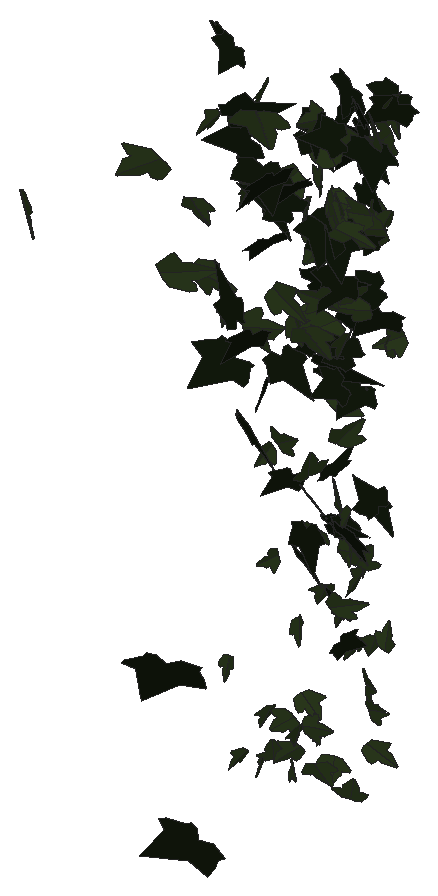
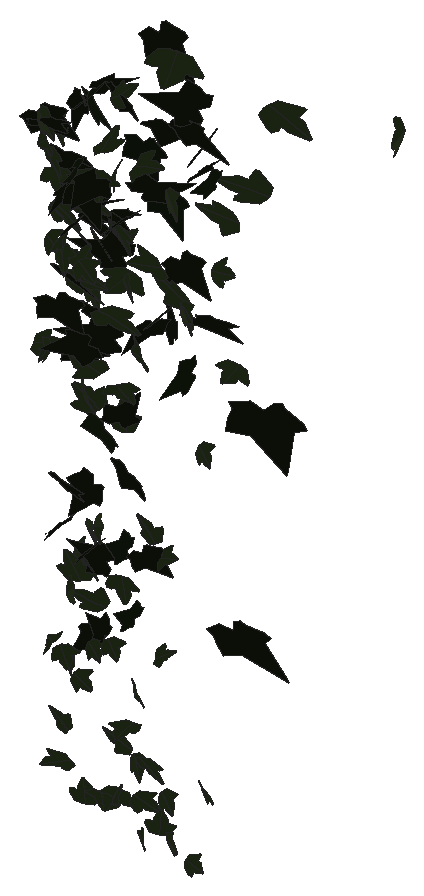
# SketchUp Ruby script. Lengths in inches.
U = 1.inch
M = Sketchup.active_model
def pt(a) = Geom::Point3d.new(a.map { |v| v * U })
def face(e, loops, mat)
  f = e.add_face(loops[0].map { |a| pt(a) })
  loops[1..].each { |l| e.add_face(l.map { |a| pt(a) }).erase! }
  f.material = f.back_material = mat if mat
  f
end
# faces: each face lists its corners as indices into pts; further lists are holes
def faces(e, pts, list, mat = nil) = list.each { |f| face(e, (f[0].is_a?(Array) ? f : [f]).map { |l| l.map { |i| pts[i] } }, mat) }
# xy, xz, yz: faces in a plane at the given z, y or x. An outline is a flat list of corners, or four numbers for a rectangle; further outlines are holes
def ring(l) = l.size == 4 ? [[l[0], l[1]], [l[2], l[1]], [l[2], l[3]], [l[0], l[3]]] : l.each_slice(2).to_a
def flat(e, list, mat, &to3) = list.each { |f| face(e, (f[0].is_a?(Array) ? f : [f]).map { |l| ring(l).map { |u, v| to3.(u, v) } }, mat) }
def xy(e, z, list, mat = nil) = flat(e, list, mat) { |x, y| [x, y, z] }
def xz(e, y, list, mat = nil) = flat(e, list, mat) { |x, z| [x, y, z] }
def yz(e, x, list, mat = nil) = flat(e, list, mat) { |y, z| [x, y, z] }
def lines(e, pts, list) = list.each { |a, b| e.add_line(pt(pts[a]), pt(pts[b])) }
# prism: a flat outline (further loops are holes) pulled along v
def prism(e, loops, v, mat = nil)
  f = face(e, loops, mat); d = Geom::Vector3d.new(v.map { |x| x * U })
  f.pushpull(f.normal.samedirection?(d) ? d.length : -d.length)
end
def box(e, o, s, mat = nil) = prism(e, [[o, [o[0] + s[0], o[1], o[2]], [o[0] + s[0], o[1] + s[1], o[2]], [o[0], o[1] + s[1], o[2]]]], [0, 0, s[2]], mat)
def at(x, y, z, deg = 0) = Geom::Transformation.translation(pt([x, y, z])) * Geom::Transformation.rotation(ORIGIN, Z_AXIS, deg.degrees)
def axes(o, x, y, z) = Geom::Transformation.new([*x, 0, *y, 0, *z, 0, *pt(o).to_a, 1])
def part(name) = M.definitions.add(name)
# library, detail: a bought-in or finely detailed component or shape, given as its bounding box
def library(name, o, s) = part(name).tap { |d| box(d.entities, o, s) }
def detail(e, o, s) = box(e.add_group.entities, o, s)
def put(e, d, t, mat = nil) = e.add_instance(d, t).tap { |i| i.material = mat if mat }
def group(e, t, mat = nil) = e.add_group.tap { |g| g.transformation = t; g.material = mat if mat }.entities
root = M.entities
M.materials.add("1026 AP 7946 SUNNY SIDE UP").color = [254, 231, 186]
M.materials.add("efeu1").color = [18, 25, 13]
M.materials.add("efeu2").color = [43, 57, 29]
c1 = part("ivyleaf_9")
p = [[1.54,2.16,1.25],[1.36,2.04,1.19],[-0.21,0.99,0.68],[-0.71,1.11,0.82],[-0.85,0.86,0.67],[-0.8,0.17,0.21],
  [-0.9,-0.01,0.1],[-0.67,-0.16,-0.02],[-0.08,-0.08,-0.05],[-0.03,-0.6,-0.4],[0.65,-0.88,-0.66],[0.83,-0.6,-0.49],
  [1.29,-0.42,-0.43],[1.8125,-0.07,-0.26],[1.21,0.44,0.15]]
faces(c1.entities,p,[[0,1,2,3,4,5,6,7,8,9,10,11,12,13,14]],"efeu1")
c2 = part("ivyleaf_10")
p = [[0,0.5,-0.03],[-0.0625,2.02,-0.43],[-0.19,2.01,-0.46],[-0.54,1.05,-0.29],[-0.52,0.625,-0.18],[-0.83,0.76,-0.28],
  [-1.16,0.64,-0.33],[-1.15,0.33,-0.24],[-0.77,-0.39,0.02],[-0.3,-0.51,0.16],[0.04,-0.48,0.23],[-0.02,2.01,-0.4375],
  [-0.06,2.01,-0.43],[0.04,-0.49,0.23],[0.67,-0.49,0.14],[1.38,0.36,-0.2],[1.375,0.51,-0.24],[0.81,0.65,-0.19],
  [0.62,0.59,-0.15],[0.6,1.09,-0.28],[0.5,1.23,-0.31]]
faces(c2.entities,p,[[0,1,2,3,4,5,6,7,8,9,10],[11,12,0,13,14,15,16,17,18,19,20]],"efeu2")
put(root,c1,axes([96.76,204.79,257.04],[0.31622,0.25415,-0.29284],[-0.24755,-0.2359,-0.34019],[-0.58798,0.236,-0.01427]),"1026 AP 7946 SUNNY SIDE UP")
put(root,c2,axes([92.11,205.87,266.17],[-0.19946,0.27307,-0.18967],[0.10139,-0.17091,-0.32043],[-0.54654,-0.13136,0.00977]),"1026 AP 7946 SUNNY SIDE UP")
put(root,c1,axes([96.56,206.05,252.18],[0.11799,0.01234,-0.4054],[-0.50602,-0.23611,-0.07008],[-0.39742,0.3043,-0.03112]),"1026 AP 7946 SUNNY SIDE UP")
put(root,c1,axes([96.82,207.04,264.5],[-0.15729,-0.25243,0.24856],[0.10943,0.22686,0.29069],[-0.57568,0.11209,-0.01265]),"1026 AP 7946 SUNNY SIDE UP")
put(root,c2,axes([93.97,207.83,266.89],[-0.32907,-0.10019,0.27299],[-0.33244,-0.17002,-0.2321],[0.32817,-0.27269,0.03861]),"1026 AP 7946 SUNNY SIDE UP")
put(root,c2,axes([94.7,207.59,264.54],[-0.15004,-0.0681,0.33403],[0.33779,0.24264,0.1201],[-0.4259,0.21643,-0.02242]),"1026 AP 7946 SUNNY SIDE UP")
put(root,c1,axes([97.24,207.8,267.68],[-0.14376,0.29444,-0.23588],[0.07304,-0.22056,-0.33064],[-0.62393,-0.09366,0.01564]),"1026 AP 7946 SUNNY SIDE UP")
put(root,c2,axes([94.8,208.48,264.21],[-0.05213,-0.01553,-0.31627],[0.4588,-0.12172,-0.02495],[-0.20331,-0.2707,0.0248]),"1026 AP 7946 SUNNY SIDE UP")
put(root,c1,axes([95.85,208.82,262.91],[-0.055,0.20258,-0.23143],[0.02728,-0.21859,-0.22226],[-0.50545,-0.03384,0.01318]),"1026 AP 7946 SUNNY SIDE UP")
put(root,c1,axes([95.07,209.17,261.92],[-0.52993,-0.11379,0.04704],[-0.05338,-0.04575,-0.35471],[0.20101,-0.31213,0.02981]),"1026 AP 7946 SUNNY SIDE UP")
put(root,c1,axes([95.87,209.09,261.23],[0.03447,0.17723,0.22376],[-0.11545,-0.1974,0.1856],[0.44754,-0.06457,0.03065]),"1026 AP 7946 SUNNY SIDE UP")
put(root,c2,axes([95.88,209.04,268.08],[-0.51085,-0.15968,-0.07554],[0.13393,-0.00356,-0.36233],[0.26277,-0.30861,0.03781]),"1026 AP 7946 SUNNY SIDE UP")
put(root,c1,axes([95.32,209.19,260.47],[0.4051,-0.21363,-0.08706],[-0.12708,0.03379,-0.34146],[0.36488,0.24895,-0.02227]),"1026 AP 7946 SUNNY SIDE UP")
put(root,c1,axes([95.69,209.4,266.63],[-0.26287,-0.20198,-0.17808],[0.20945,0.11062,-0.26953],[0.38847,-0.19632,0.02482]),"1026 AP 7946 SUNNY SIDE UP")
put(root,c2,axes([95.26,209.61,262.56],[0.21015,-0.10079,-0.30372],[0.41701,-0.14108,0.16723],[-0.29184,-0.27416,0.02025]),"1026 AP 7946 SUNNY SIDE UP")
put(root,c1,axes([95.75,209.48,264.89],[-0.01144,0.27838,-0.10004],[0.00367,-0.09705,-0.29947],[-0.50045,-0.00708,0.00009]),"1026 AP 7946 SUNNY SIDE UP")
put(root,c1,axes([95.07,209.6875,266.99],[-0.01867,-0.04256,-0.3261],[-0.49086,-0.10081,0.0249],[-0.17514,0.28706,-0.03501]),"1026 AP 7946 SUNNY SIDE UP")
put(root,c1,axes([94.79,209.64,267.48],[0.11811,0.04297,0.35046],[0.5169,0.1195,-0.08455],[-0.21422,0.31202,-0.0108]),"1026 AP 7946 SUNNY SIDE UP")
put(root,c1,axes([96.46,209.9375,257.91],[-0.26713,-0.0282,-0.2717],[0.43281,-0.01369,-0.16806],[0.0054,-0.29798,0.02923]),"1026 AP 7946 SUNNY SIDE UP")
put(root,c2,axes([96.79,210.02,263.57],[-0.12681,-0.0987,-0.24808],[-0.24998,-0.17731,0.12994],[-0.34438,0.16505,-0.00298]),"1026 AP 7946 SUNNY SIDE UP")
put(root,c1,axes([96.125,209.78,266.18],[0.03002,0.28231,-0.07055],[-0.00699,-0.06946,-0.30379],[-0.49352,0.01815,0.00001]),"1026 AP 7946 SUNNY SIDE UP")
put(root,c2,axes([95.69,209.92,263.35],[0.22264,0.02384,0.28435],[0.45215,-0.01413,-0.13981],[0.00365,0.29561,-0.02545]),"1026 AP 7946 SUNNY SIDE UP")
put(root,c2,axes([96.58,209.85,262.76],[-0.39525,-0.05768,-0.14847],[0.23823,0.00369,-0.25522],[0.0875,-0.2706,0.02422]),"1026 AP 7946 SUNNY SIDE UP")
put(root,c2,axes([96.41,210.09,259.24],[-0.13203,-0.27231,-0.09841],[-0.03041,-0.08677,0.3019],[-0.48504,0.07956,0.00786]),"1026 AP 7946 SUNNY SIDE UP")
put(root,c1,axes([95.8,209.94,261.85],[0.09352,-0.22709,-0.23612],[-0.06194,0.2148,-0.24689],[0.53029,0.06514,0.01281]),"1026 AP 7946 SUNNY SIDE UP")
put(root,c1,axes([97.09,210.2,267.47],[-0.20282,-0.05341,0.25391],[-0.29832,-0.16473,-0.1364],[0.28683,-0.20909,0.03768]),"1026 AP 7946 SUNNY SIDE UP")
put(root,c1,axes([97.07,210.28,261.49],[-0.18841,-0.12241,0.2142],[-0.16462,-0.1795,-0.17628],[0.36507,-0.14412,0.03106]),"1026 AP 7946 SUNNY SIDE UP")
put(root,c1,axes([95.76,210.1875,265.31],[-0.07196,0.0321,0.30452],[-0.48333,-0.03002,-0.04228],[0.04272,-0.2856,0.03459]),"1026 AP 7946 SUNNY SIDE UP")
put(root,c2,axes([95.77,210.35,266.05],[0.12707,0.12283,-0.29191],[-0.1913,-0.25055,-0.15655],[-0.47291,0.13435,-0.01511]),"1026 AP 7946 SUNNY SIDE UP")
put(root,c1,axes([97.15,210.27,264.12],[-0.47959,-0.0158,-0.11049],[0.17622,-0.01682,-0.30232],[0.01536,-0.30024,0.01853]),"1026 AP 7946 SUNNY SIDE UP")
put(root,c2,axes([96.33,210.43,267.59],[-0.02492,0.05935,0.29452],[0.05971,-0.27215,0.06125],[0.47271,0.03751,0.00779]),"1026 AP 7946 SUNNY SIDE UP")
put(root,c1,axes([96.32,210.4,267.64],[-0.29082,-0.01958,-0.23941],[0.38013,-0.0293,-0.18153],[-0.01944,-0.27997,0.03177]),"1026 AP 7946 SUNNY SIDE UP")
put(root,c2,axes([96.66,210.43,263.54],[0.18759,-0.1561,-0.17936],[0.20715,-0.11461,0.20137],[-0.32595,-0.16268,0.02475]),"1026 AP 7946 SUNNY SIDE UP")
put(root,c2,axes([97.09,210.45,262.6],[0.00771,-0.26051,0.02821],[0.00502,-0.0297,-0.27934],[0.44507,0.00485,0.00266]),"1026 AP 7946 SUNNY SIDE UP")
put(root,c1,axes([96.59,210.64,264.76],[-0.28307,-0.1446,-0.2224],[0.37207,0.0377,-0.21791],[0.2096,-0.26222,0.08646]),"1026 AP 7946 SUNNY SIDE UP")
put(root,c1,axes([96.27,210.44,263.65],[0.16696,0.01748,0.27789],[0.44123,-0.0051,-0.10523],[-0.00241,0.27732,-0.01557]),"1026 AP 7946 SUNNY SIDE UP")
put(root,c1,axes([96.35,210.7,264.8],[-0.24627,-0.23153,-0.02228],[0.03909,0.00653,-0.29192],[0.39226,-0.14601,0.01511]),"1026 AP 7946 SUNNY SIDE UP")
put(root,c1,axes([97.1,210.59,262.07],[-0.35743,-0.08481,-0.12875],[-0.19987,-0.02563,0.2419],[-0.1473,0.24057,-0.0158]),"1026 AP 7946 SUNNY SIDE UP")
put(root,c2,axes([96.22,210.65,264.47],[0.3782,-0.18524,-0.05736],[-0.09213,0.01449,-0.30899],[0.31295,0.22813,-0.02165]),"1026 AP 7946 SUNNY SIDE UP")
put(root,c1,axes([96.42,210.56,261.57],[0.31632,0.01269,0.2436],[0.38523,-0.03481,-0.19752],[0.03219,0.29191,-0.03]),"1026 AP 7946 SUNNY SIDE UP")
put(root,c1,axes([96.92,210.625,257.76],[0.44751,-0.04637,-0.10647],[-0.1705,-0.00169,-0.28594],[0.07268,0.28154,-0.01522]),"1026 AP 7946 SUNNY SIDE UP")
put(root,c2,axes([96.89,210.61,264.99],[-0.18325,-0.10283,-0.23851],[0.34983,0.09147,-0.15174],[0.22227,-0.22874,0.04219]),"1026 AP 7946 SUNNY SIDE UP")
put(root,c1,axes([96.7,210.49,259.17],[-0.2338,0.23128,-0.1163],[-0.07387,0.10384,0.28921],[0.42966,0.1437,-0.01356]),"1026 AP 7946 SUNNY SIDE UP")
put(root,c2,axes([97.01,210.89,263.4],[-0.12961,-0.16832,-0.16863],[-0.12959,-0.13566,0.19567],[-0.36657,0.10747,-0.00955]),"1026 AP 7946 SUNNY SIDE UP")
put(root,c1,axes([96.64,210.98,265.02],[-0.23121,-0.26511,0.07266],[0.05058,-0.09343,-0.31215],[0.46328,-0.12211,0.07034]),"1026 AP 7946 SUNNY SIDE UP")
put(root,c2,axes([96.58,210.69,265.33],[-0.02008,0.24122,0.08878],[-0.02199,0.07919,-0.25728],[-0.43073,-0.01529,0.009]),"1026 AP 7946 SUNNY SIDE UP")
put(root,c1,axes([97.03,210.97,261.13],[-0.31101,-0.19534,0.03687],[-0.02075,-0.03913,-0.28663],[0.33685,-0.18276,0.01638]),"1026 AP 7946 SUNNY SIDE UP")
put(root,c2,axes([96.78,210.73,259.89],[-0.15602,-0.22079,0.1488],[0.07236,0.13576,0.25766],[-0.43959,0.10071,-0.0104]),"1026 AP 7946 SUNNY SIDE UP")
put(root,c2,axes([96.75,210.71,260.72],[0.26225,0.07892,-0.21619],[0.28132,0.11885,0.18617],[0.23983,-0.2257,0.01803]),"1026 AP 7946 SUNNY SIDE UP")
put(root,c2,axes([96.23,210.93,262.41],[0.35497,0.029,-0.22598],[-0.34037,-0.07477,-0.2243],[-0.12419,0.28784,-0.03117]),"1026 AP 7946 SUNNY SIDE UP")
put(root,c2,axes([96.36,210.84,266.49],[0.08365,0.28964,0.04034],[-0.02287,-0.03209,0.31397],[0.4945,-0.05048,0.0077]),"1026 AP 7946 SUNNY SIDE UP")
put(root,c2,axes([96.47,210.85,265.54],[-0.00074,0.31146,-0.03662],[0.00224,-0.03826,-0.33397],[-0.53268,-0.0006,-0.00136]),"1026 AP 7946 SUNNY SIDE UP")
put(root,c2,axes([96.19,210.66,265.87],[0.00823,0.08522,-0.28036],[-0.04237,0.26209,0.09408],[0.46737,0.02226,0.01347]),"1026 AP 7946 SUNNY SIDE UP")
put(root,c2,axes([96.49,210.88,265.47],[0.09882,0.3056,-0.027],[0.0015,-0.0299,-0.3334],[-0.52113,0.05786,-0.00608]),"1026 AP 7946 SUNNY SIDE UP")
put(root,c2,axes([97.11,210.98,263.02],[-0.07467,0.00165,0.25011],[-0.32064,-0.14011,-0.03897],[0.23333,-0.19202,0.02648]),"1026 AP 7946 SUNNY SIDE UP")
put(root,c1,axes([96.68,211.06,267.6875],[-0.33881,0.13455,-0.17552],[0.20651,-0.1147,-0.25819],[-0.29773,-0.23267,0.02065]),"1026 AP 7946 SUNNY SIDE UP")
put(root,c2,axes([96.37,211,265.45],[-0.26332,0.25966,-0.05872],[0.02425,-0.05918,-0.32408],[-0.45108,-0.15476,0.01685]),"1026 AP 7946 SUNNY SIDE UP")
put(root,c2,axes([96.8,211.22,256.36],[0.0399,-0.09067,0.2451],[0.12446,-0.22498,-0.09813],[0.3813,0.08292,0.00638]),"1026 AP 7946 SUNNY SIDE UP")
put(root,c2,axes([95.02,211.27,261.91],[0.17616,-0.04264,0.27108],[0.34964,-0.15024,-0.1193],[0.26182,0.22933,-0.02308]),"1026 AP 7946 SUNNY SIDE UP")
put(root,c2,axes([96.96,211.13,265.21],[0.13555,-0.01949,-0.28992],[-0.44932,0.05607,-0.08718],[0.10068,0.27646,0.00128]),"1026 AP 7946 SUNNY SIDE UP")
put(root,c1,axes([96.45,211.4375,267.92],[-0.07216,-0.22327,0.20327],[-0.03762,-0.19181,-0.24572],[0.49933,-0.04671,0.01086]),"1026 AP 7946 SUNNY SIDE UP")
put(root,c1,axes([97.32,211.2,264.66],[-0.24554,0.17419,0.07781],[-0.09921,0.04273,-0.24113],[-0.30311,-0.15509,0.01589]),"1026 AP 7946 SUNNY SIDE UP")
put(root,c1,axes([96.75,211.22,267.74],[0.29223,-0.05908,-0.19794],[-0.30059,0.05088,-0.19401],[0.13188,0.24688,-0.00359]),"1026 AP 7946 SUNNY SIDE UP")
put(root,c2,axes([97.3125,211.3,264.88],[-0.19055,0.04583,0.23418],[-0.37648,0.00157,-0.12251],[-0.03801,-0.24533,0.03942]),"1026 AP 7946 SUNNY SIDE UP")
put(root,c1,axes([97.18,211.37,263.37],[-0.4502,0.1023,0.03345],[-0.06098,-0.01027,-0.30351],[-0.17034,-0.26669,0.02024]),"1026 AP 7946 SUNNY SIDE UP")
put(root,c2,axes([96.84,211.47,253.64],[-0.12272,0.07005,0.23584],[0.30166,-0.12505,0.10625],[0.2242,0.20659,-0.01387]),"1026 AP 7946 SUNNY SIDE UP")
put(root,c2,axes([95.34,211.43,252.14],[0.09559,-0.05032,-0.22976],[0.31746,-0.09584,0.07852],[-0.16776,-0.21005,0.01766]),"1026 AP 7946 SUNNY SIDE UP")
put(root,c2,axes([96.18,211.32,255.36],[-0.15734,-0.06078,0.22516],[0.25434,0.14891,0.11963],[-0.25084,0.1891,-0.01993]),"1026 AP 7946 SUNNY SIDE UP")
put(root,c1,axes([96.32,211.29,254.59],[-0.01301,0.02501,-0.25525],[-0.13285,0.23307,0.02849],[0.36858,0.08489,0.00126]),"1026 AP 7946 SUNNY SIDE UP")
put(root,c2,axes([94.98,211.5,251.94],[-0.00745,-0.23171,-0.01564],[0.00479,0.01381,-0.23866],[0.36496,-0.00491,0.00282]),"1026 AP 7946 SUNNY SIDE UP")
put(root,c1,axes([97.15,211.55,262.69],[0.11918,0.13233,-0.24427],[-0.14865,-0.21292,-0.16281],[-0.42505,0.11157,-0.01155]),"1026 AP 7946 SUNNY SIDE UP")
put(root,c1,axes([97.125,211.44,258.11],[-0.33665,0.00804,-0.15131],[-0.22838,0.02999,0.21991],[0.03705,0.25792,-0.01933]),"1026 AP 7946 SUNNY SIDE UP")
put(root,c1,axes([96.85,211.64,266.54],[-0.33708,-0.13563,-0.16656],[0.24213,0.06248,-0.25525],[0.25011,-0.24328,0.02263]),"1026 AP 7946 SUNNY SIDE UP")
put(root,c2,axes([94.65,211.57,252.02],[0.2905,-0.07094,-0.1166],[-0.17836,0.0174,-0.2026],[0.10991,0.21576,-0.02059]),"1026 AP 7946 SUNNY SIDE UP")
put(root,c2,axes([97.21,211.38,266.99],[-0.07274,0.09334,-0.27361],[-0.18286,0.2331,0.1132],[0.42624,0.11593,0.00187]),"1026 AP 7946 SUNNY SIDE UP")
put(root,c2,axes([96.21,211.7,260.7],[0.23048,-0.12885,0.19348],[0.19047,-0.14606,-0.2007],[0.30441,0.18895,-0.02092]),"1026 AP 7946 SUNNY SIDE UP")
put(root,c2,axes([95.17,211.49,252.73],[0.16574,0.18338,0.10562],[0.09705,0.0814,-0.2171],[-0.31495,0.12159,-0.01131]),"1026 AP 7946 SUNNY SIDE UP")
put(root,c2,axes([96.125,211.6875,257.42],[0.19705,-0.2116,0.02366],[0.00282,-0.02699,-0.2532],[0.33488,0.12474,-0.01179]),"1026 AP 7946 SUNNY SIDE UP")
put(root,c2,axes([94.65,211.78,251.2],[-0.13826,-0.11587,0.17426],[-0.10854,-0.15733,-0.14834],[0.30448,-0.1087,0.02625]),"1026 AP 7946 SUNNY SIDE UP")
put(root,c1,axes([92.93,211.87,267.51],[-0.11246,-0.20782,0.14205],[-0.06539,-0.13275,-0.22718],[0.38773,-0.08267,0.00289]),"1026 AP 7946 SUNNY SIDE UP")
put(root,c2,axes([96.21,211.73,250.65],[-0.30519,-0.08983,0.00949],[0.00726,0.01315,0.22017],[-0.14188,0.19389,-0.00915]),"1026 AP 7946 SUNNY SIDE UP")
put(root,c2,axes([95.36,211.6875,251.05],[-0.28738,-0.10428,-0.09434],[0.13639,0.03111,-0.21607],[0.16956,-0.20177,0.01392]),"1026 AP 7946 SUNNY SIDE UP")
put(root,c1,axes([95.59,211.89,255.06],[0.10301,-0.11211,0.21471],[0.119,-0.19567,-0.13367],[0.35351,0.09853,-0.01757]),"1026 AP 7946 SUNNY SIDE UP")
put(root,c1,axes([94.97,211.87,257.37],[0.22261,-0.17413,0.11388],[0.08929,-0.09724,-0.23121],[0.31265,0.15175,-0.01506]),"1026 AP 7946 SUNNY SIDE UP")
put(root,c2,axes([95.97,211.9,256.65],[0.23883,-0.09291,0.18691],[0.21845,-0.11928,-0.18291],[0.23555,0.20482,-0.01988]),"1026 AP 7946 SUNNY SIDE UP")
put(root,c1,axes([95.91,211.88,257.08],[0.11336,-0.23682,-0.0694],[-0.0355,0.06213,-0.25464],[0.38495,0.07547,-0.00305]),"1026 AP 7946 SUNNY SIDE UP")
put(root,c2,axes([96.33,211.84,256.28],[-0.33745,-0.11311,0.08436],[0.09928,0.05663,0.24943],[-0.19651,0.22284,-0.01885]),"1026 AP 7946 SUNNY SIDE UP")
put(root,c1,axes([94.67,211.97,255.8],[0.16559,-0.19279,0.10222],[0.07376,-0.08868,-0.22682],[0.33367,0.11528,-0.00059]),"1026 AP 7946 SUNNY SIDE UP")
put(root,c2,axes([93.98,211.92,250.74],[-0.205,-0.16585,-0.04292],[-0.05523,-0.02409,0.21681],[-0.26279,0.13445,-0.01208]),"1026 AP 7946 SUNNY SIDE UP")
put(root,c1,axes([97.23,211.99,267.56],[0.03011,0.05998,-0.28282],[-0.11576,-0.25604,-0.07052],[-0.44639,0.07044,-0.00079]),"1026 AP 7946 SUNNY SIDE UP")
put(root,c2,axes([93.65,211.98,250.57],[0.14133,-0.15974,0.10656],[0.06167,-0.09741,-0.189],[0.29361,0.09735,-0.0116]),"1026 AP 7946 SUNNY SIDE UP")
put(root,c1,axes([95.54,211.89,256.89],[0.26716,0.02416,-0.19098],[0.27346,0.07196,0.17416],[0.10842,-0.24105,0.0313]),"1026 AP 7946 SUNNY SIDE UP")
put(root,c2,axes([95.875,211.74,257.58],[-0.09561,0.10975,-0.21482],[-0.13571,0.19071,0.13006],[0.34572,0.10522,-0.00836]),"1026 AP 7946 SUNNY SIDE UP")
put(root,c2,axes([95.07,211.91,256.56],[-0.35446,0.00293,0.06171],[-0.09394,-0.03065,-0.23031],[0.00796,-0.23122,0.02994]),"1026 AP 7946 SUNNY SIDE UP")
put(root,c2,axes([97.21,212.09,261.88],[0.08603,0.03927,-0.2571],[-0.2261,-0.20539,-0.06691],[-0.32704,0.15232,-0.02137]),"1026 AP 7946 SUNNY SIDE UP")
put(root,c2,axes([95.8125,211.96,266.47],[-0.41858,-0.10135,0.06033],[-0.06201,-0.06097,-0.28278],[0.18799,-0.24578,0.04105]),"1026 AP 7946 SUNNY SIDE UP")
put(root,c1,axes([94.32,212.05,257.58],[-0.00429,0.08886,-0.23244],[-0.02938,-0.22555,-0.0924],[-0.3809,0.0164,0.00974]),"1026 AP 7946 SUNNY SIDE UP")
put(root,c2,axes([93.625,212.02,266.73],[0.08552,-0.25123,0.00762],[-0.00201,-0.0093,-0.26485],[0.39528,0.05431,-0.00299]),"1026 AP 7946 SUNNY SIDE UP")
put(root,c2,axes([95.49,212.01,251.09],[0.33656,0.02654,0.02645],[0.04347,-0.01642,-0.22137],[-0.03824,0.21493,-0.01889]),"1026 AP 7946 SUNNY SIDE UP")
put(root,c2,axes([92.17,212.16,265.43],[0.031,-0.115,0.22397],[0.02669,-0.2176,-0.12107],[0.38671,0.02424,-0.0096]),"1026 AP 7946 SUNNY SIDE UP")
put(root,c2,axes([94.46,212.1,254.04],[0.19238,-0.08379,0.18368],[0.2115,-0.11858,-0.15279],[0.22726,0.18129,-0.0133]),"1026 AP 7946 SUNNY SIDE UP")
put(root,c2,axes([92.96,212.125,250.35],[-0.00557,-0.14778,0.14293],[-0.00061,-0.1396,-0.15309],[0.31964,-0.00284,0.0022]),"1026 AP 7946 SUNNY SIDE UP")
put(root,c2,axes([93.72,212.07,251.7],[-0.02684,-0.20834,0.05577],[-0.00474,-0.05526,-0.21567],[0.33892,-0.01727,0.0014]),"1026 AP 7946 SUNNY SIDE UP")
put(root,c2,axes([95.95,212.15,264.25],[-0.12599,-0.19384,0.11935],[-0.01953,-0.12011,-0.21455],[0.35544,-0.07531,0.03052]),"1026 AP 7946 SUNNY SIDE UP")
put(root,c1,axes([96.04,212.01,266.05],[0.0564,0.23522,-0.13262],[-0.05552,-0.12338,-0.25564],[-0.45033,0.04467,0.01491]),"1026 AP 7946 SUNNY SIDE UP")
put(root,c2,axes([95.71,212.13,254.8],[-0.03097,-0.18887,0.07854],[0.00947,-0.07818,-0.19563],[0.32076,-0.01593,0.01336]),"1026 AP 7946 SUNNY SIDE UP")
put(root,c2,axes([94.25,212.17,250.43],[0.013,0.01026,0.20843],[0.24146,-0.1323,-0.00032],[0.20762,0.15322,-0.01267]),"1026 AP 7946 SUNNY SIDE UP")
put(root,c2,axes([96.56,212.1,254.39],[-0.17455,-0.16804,0.04654],[-0.01892,-0.04718,-0.20713],[0.27334,-0.11057,0.01539]),"1026 AP 7946 SUNNY SIDE UP")
put(root,c2,axes([97.0625,212.15,267.59],[0.06247,-0.2586,0.0719],[0.00087,-0.07112,-0.28046],[0.45501,0.03564,-0.00934]),"1026 AP 7946 SUNNY SIDE UP")
put(root,c2,axes([96.8125,212.2,264.64],[-0.01657,-0.19811,0.144],[0.06837,-0.1403,-0.20068],[0.37609,0.01677,0.04283]),"1026 AP 7946 SUNNY SIDE UP")
put(root,c2,axes([93.11,212.14,264.13],[0.08157,-0.23182,0.05317],[0.01863,-0.05159,-0.24503],[0.37344,0.05321,0.00061]),"1026 AP 7946 SUNNY SIDE UP")
put(root,c1,axes([96.03,211.94,262.16],[0.06069,0.05378,-0.26669],[0.18394,0.23149,0.06879],[0.37337,-0.12278,0.00946]),"1026 AP 7946 SUNNY SIDE UP")
put(root,c2,axes([94.67,212.19,264.22],[0.18218,-0.18488,0.1186],[0.10682,-0.09447,-0.22522],[0.32629,0.13415,0.00751]),"1026 AP 7946 SUNNY SIDE UP")
put(root,c1,axes([92.28,212.16,267.61],[0.24464,-0.20369,0.01249],[-0.0059,-0.01955,-0.26372],[0.3209,0.15492,-0.01437]),"1026 AP 7946 SUNNY SIDE UP")
put(root,c2,axes([93.73,212.25,255.3],[0.03244,0.01868,-0.2195],[-0.1279,-0.19741,-0.02708],[-0.31123,0.08307,-0.01175]),"1026 AP 7946 SUNNY SIDE UP")
put(root,c1,axes([94.9,212.19,260.78],[0.14585,0.06554,0.23065],[-0.33391,-0.07505,0.11302],[0.15048,-0.23006,0.02724]),"1026 AP 7946 SUNNY SIDE UP")
put(root,c2,axes([96.43,212.16,252.58],[-0.15837,0.04715,0.19973],[0.30056,-0.03846,0.11186],[0.08856,0.21483,-0.02245]),"1026 AP 7946 SUNNY SIDE UP")
put(root,c2,axes([96.93,212.0625,266.72],[0.24278,-0.13804,-0.15105],[-0.13448,0.12124,-0.2108],[0.28569,0.17438,0.02914]),"1026 AP 7946 SUNNY SIDE UP")
put(root,c2,axes([93.13,212.12,264.09],[0.22642,-0.18941,-0.0543],[-0.03342,0.04861,-0.24451],[0.30689,0.14504,0.01344]),"1026 AP 7946 SUNNY SIDE UP")
put(root,c2,axes([96.2,212.29,256.0625],[0.06269,-0.02943,0.23614],[0.1903,-0.1957,-0.04868],[0.30987,0.12613,-0.01788]),"1026 AP 7946 SUNNY SIDE UP")
put(root,c2,axes([93.58,212.26,257.84],[0.05324,0.11144,-0.20584],[-0.09601,-0.19092,-0.12109],[-0.3476,0.0698,0.00192]),"1026 AP 7946 SUNNY SIDE UP")
put(root,c2,axes([97.07,211.95,261.73],[-0.00181,0.03529,0.25164],[-0.14011,0.21988,-0.03274],[-0.37754,-0.08177,0.01094]),"1026 AP 7946 SUNNY SIDE UP")
put(root,c2,axes([96.54,212.12,264.41],[-0.01966,-0.24613,-0.05539],[0.0189,0.04803,-0.26296],[0.42545,-0.01351,0.00912]),"1026 AP 7946 SUNNY SIDE UP")
put(root,c2,axes([96.91,211.99,254.43],[0.06158,0.16442,-0.16566],[0.01518,0.16275,0.17379],[0.36234,-0.03476,0.02087]),"1026 AP 7946 SUNNY SIDE UP")
put(root,c2,axes([95.15,212.19,255.1],[-0.11002,-0.18275,0.05203],[-0.02021,-0.05025,-0.20181],[0.29789,-0.07091,0.00553]),"1026 AP 7946 SUNNY SIDE UP")
put(root,c1,axes([94.73,212.14,265.87],[0.13735,-0.21244,-0.11502],[-0.00994,0.11548,-0.2333],[0.37635,0.08058,0.03581]),"1026 AP 7946 SUNNY SIDE UP")
put(root,c2,axes([96.5,212.18,264.77],[-0.00242,0.24386,-0.08272],[-0.02351,-0.0804,-0.26179],[-0.43526,0.00299,0.0146]),"1026 AP 7946 SUNNY SIDE UP")
put(root,c1,axes([95.7,212.03,266.47],[0.43193,0.08296,-0.05266],[-0.0926,0.00568,-0.28547],[-0.13616,0.2593,0.02709]),"1026 AP 7946 SUNNY SIDE UP")
put(root,c1,axes([96.98,212.3,267.6],[-0.32542,-0.14515,0.03944],[-0.03025,-0.04043,-0.25969],[0.23444,-0.2067,0.02124]),"1026 AP 7946 SUNNY SIDE UP")
put(root,c1,axes([96.24,212.12,265.18],[0.16149,-0.17898,-0.1373],[-0.09169,0.11894,-0.21176],[0.33771,0.11788,0.00816]),"1026 AP 7946 SUNNY SIDE UP")
put(root,c2,axes([94.85,212.21,261.61],[0.30758,0.10907,-0.1041],[-0.12156,-0.06922,-0.23014],[-0.20049,0.20931,-0.02017]),"1026 AP 7946 SUNNY SIDE UP")
put(root,c2,axes([93.95,212.18,258.17],[-0.25662,0.03249,0.17428],[0.26629,-0.01101,0.17061],[0.04802,0.23467,-0.01472]),"1026 AP 7946 SUNNY SIDE UP")
put(root,c2,axes([96.63,212.17,266.34],[-0.36366,-0.08472,0.04733],[-0.05687,-0.03575,-0.25305],[0.14085,-0.23317,0.02003]),"1026 AP 7946 SUNNY SIDE UP")
put(root,c1,axes([96.1,212.18,266.63],[0.23961,-0.20373,-0.06768],[-0.08359,0.04064,-0.26122],[0.32547,0.16042,-0.01726]),"1026 AP 7946 SUNNY SIDE UP")
put(root,c2,axes([92.48,212.24,252.37],[0.23636,-0.11626,0.08573],[0.08854,-0.06388,-0.19556],[0.2073,0.15984,-0.01422]),"1026 AP 7946 SUNNY SIDE UP")
put(root,c1,axes([93.6875,212.2,263.83],[0.14654,-0.21701,-0.06035],[-0.03052,0.05407,-0.24296],[0.35161,0.09514,0.00406]),"1026 AP 7946 SUNNY SIDE UP")
put(root,c2,axes([91.67,212.16,263.18],[-0.34239,0.00795,-0.09259],[0.13938,-0.02563,-0.22361],[-0.02687,-0.23419,0.01994]),"1026 AP 7946 SUNNY SIDE UP")
put(root,c1,axes([96.35,212.12,266.09],[0.10356,-0.1734,-0.20455],[-0.13742,0.17112,-0.19386],[0.4129,0.10044,-0.01322]),"1026 AP 7946 SUNNY SIDE UP")
put(root,c2,axes([95.96,212.29,254.01],[-0.05394,-0.17102,0.12959],[-0.02728,-0.12572,-0.18032],[0.33362,-0.03793,0.0062]),"1026 AP 7946 SUNNY SIDE UP")
put(root,c2,axes([96.86,212.29,267.12],[0.20187,-0.09141,0.20387],[0.27179,-0.09823,-0.16242],[0.21006,0.21494,0.01422]),"1026 AP 7946 SUNNY SIDE UP")
put(root,c1,axes([96.48,212.22,257.65],[0.102,-0.22126,-0.07916],[-0.03161,0.07287,-0.2371],[0.36628,0.0679,0.00158]),"1026 AP 7946 SUNNY SIDE UP")
put(root,c2,axes([96.47,212.14,251.69],[0.15999,0.08268,0.19339],[0.26359,0.08634,-0.13261],[-0.1847,0.19484,-0.02173]),"1026 AP 7946 SUNNY SIDE UP")
put(root,c2,axes([92.5,212.29,260.9],[-0.00847,-0.21134,0.07951],[0.02376,-0.07857,-0.21762],[0.35363,0.00022,0.01653]),"1026 AP 7946 SUNNY SIDE UP")
put(root,c2,axes([94.86,212.35,251.43],[-0.06348,0.02398,0.20727],[0.14102,-0.1817,0.03981],[0.28546,0.09509,0.02642]),"1026 AP 7946 SUNNY SIDE UP")
